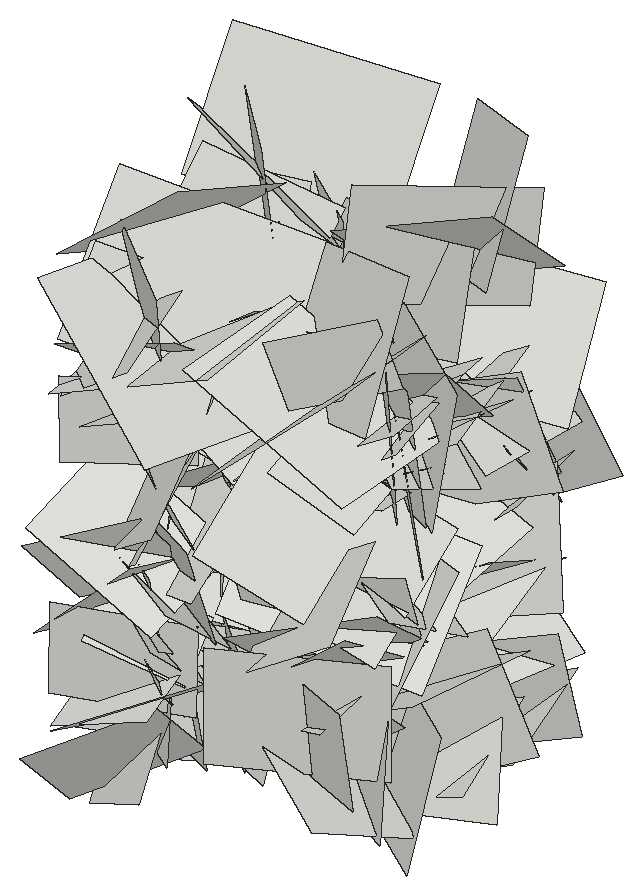
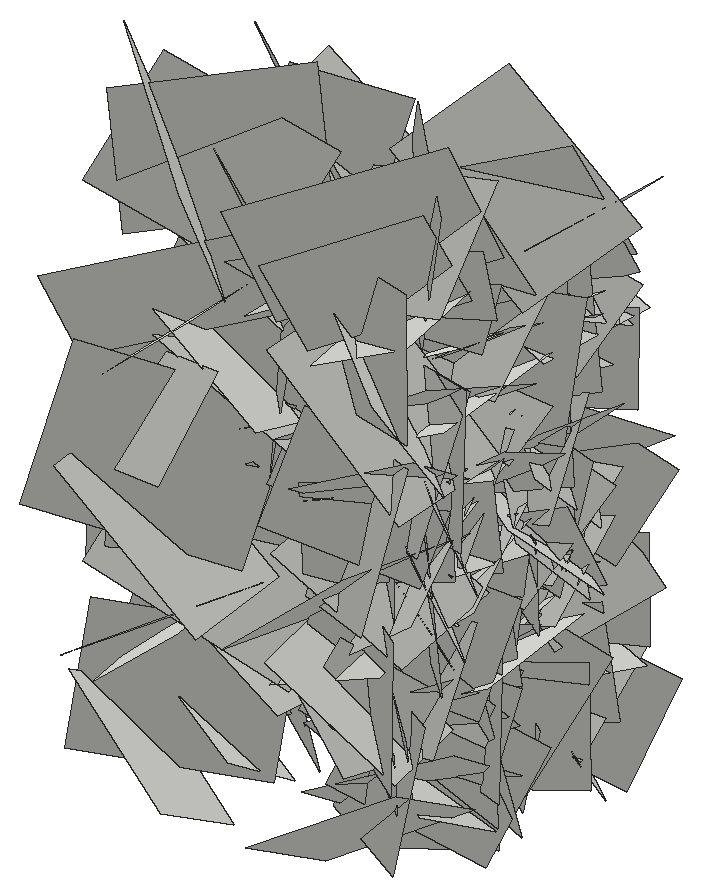
# SketchUp Ruby script. Lengths in inches.
U = 1.inch
M = Sketchup.active_model
def pt(a) = Geom::Point3d.new(a.map { |v| v * U })
def face(e, loops, mat)
  f = e.add_face(loops[0].map { |a| pt(a) })
  loops[1..].each { |l| e.add_face(l.map { |a| pt(a) }).erase! }
  f.material = f.back_material = mat if mat
  f
end
# faces: each face lists its corners as indices into pts; further lists are holes
def faces(e, pts, list, mat = nil) = list.each { |f| face(e, (f[0].is_a?(Array) ? f : [f]).map { |l| l.map { |i| pts[i] } }, mat) }
# xy, xz, yz: faces in a plane at the given z, y or x. An outline is a flat list of corners, or four numbers for a rectangle; further outlines are holes
def ring(l) = l.size == 4 ? [[l[0], l[1]], [l[2], l[1]], [l[2], l[3]], [l[0], l[3]]] : l.each_slice(2).to_a
def flat(e, list, mat, &to3) = list.each { |f| face(e, (f[0].is_a?(Array) ? f : [f]).map { |l| ring(l).map { |u, v| to3.(u, v) } }, mat) }
def xy(e, z, list, mat = nil) = flat(e, list, mat) { |x, y| [x, y, z] }
def xz(e, y, list, mat = nil) = flat(e, list, mat) { |x, z| [x, y, z] }
def yz(e, x, list, mat = nil) = flat(e, list, mat) { |y, z| [x, y, z] }
def lines(e, pts, list) = list.each { |a, b| e.add_line(pt(pts[a]), pt(pts[b])) }
# prism: a flat outline (further loops are holes) pulled along v
def prism(e, loops, v, mat = nil)
  f = face(e, loops, mat); d = Geom::Vector3d.new(v.map { |x| x * U })
  f.pushpull(f.normal.samedirection?(d) ? d.length : -d.length)
end
def box(e, o, s, mat = nil) = prism(e, [[o, [o[0] + s[0], o[1], o[2]], [o[0] + s[0], o[1] + s[1], o[2]], [o[0], o[1] + s[1], o[2]]]], [0, 0, s[2]], mat)
def at(x, y, z, deg = 0) = Geom::Transformation.translation(pt([x, y, z])) * Geom::Transformation.rotation(ORIGIN, Z_AXIS, deg.degrees)
def axes(o, x, y, z) = Geom::Transformation.new([*x, 0, *y, 0, *z, 0, *pt(o).to_a, 1])
def part(name) = M.definitions.add(name)
# library, detail: a bought-in or finely detailed component or shape, given as its bounding box
def library(name, o, s) = part(name).tap { |d| box(d.entities, o, s) }
def detail(e, o, s) = box(e.add_group.entities, o, s)
def put(e, d, t, mat = nil) = e.add_instance(d, t).tap { |i| i.material = mat if mat }
def group(e, t, mat = nil) = e.add_group.tap { |g| g.transformation = t; g.material = mat if mat }.entities
root = M.entities
c1 = part("Component\#6")
p = [[0.01,0,0],[0,3.24,4.54],[4.32,3.24,4.54],[4.33,0,0]]
faces(c1.entities,p,[[0,1,2,3]])
put(root,c1,axes([28.31,154.27,5.56],[0.10843,0.64197,-0.78685],[0.13439,-0.79271,-0.63027],[-1.06801,-0.03458,-0.15919]))
put(root,c1,axes([24.34,149.67,1.32],[0.10197,-0.47157,-0.58691],[-0.00963,-0.59236,0.47447],[0.798,0.05311,0.08072]))
put(root,c1,axes([24.34,151.77,10.3],[0.00621,-0.04081,-0.81439],[0.02737,-0.814,0.04098],[0.86391,0.02608,0.00455]))
put(root,c1,axes([28.31,158.76,13.54],[0.17018,-0.33172,-0.9968],[0.1229,-0.99662,0.35033],[-1.10678,-0.16167,-0.11436]))
put(root,c1,axes([24.34,155.14,21.07],[-0.01676,0.7943,-0.14622],[0.08914,-0.14383,-0.79043],[0.85145,0.03069,0.07988]))
put(root,c1,axes([28.31,152.55,8.85],[0.17208,0.39932,0.93109],[0.08126,0.93542,-0.41455],[-1.07081,0.13515,0.11817]))
put(root,c1,axes([24.34,155.22,14.18],[-0.0107,0.67836,0.43703],[0.08223,0.43585,-0.67474],[0.8514,-0.03357,0.07066]))
put(root,c1,axes([28.31,154.72,7.86],[-0.01434,-0.12328,-0.7123],[-0.10241,-0.70572,0.12398],[-0.75939,0.0975,-0.00327]))
put(root,c1,axes([24.34,153.88,7.81],[0.12498,-0.19712,-0.75186],[-0.05107,-0.76085,0.19192],[0.82232,-0.01729,0.12619]))
put(root,c1,axes([28.31,156.49,11.61],[0.16435,-0.92659,-0.48849],[0.14398,-0.47186,0.93815],[-1.10094,-0.20004,0.04977]))
put(root,c1,axes([28.31,155.82,10.86],[0.10869,-0.77244,0.23734],[-0.13092,0.22145,0.77409],[-0.8465,-0.13343,-0.08925]))
put(root,c1,axes([24.34,152.8,10.75],[-0.04843,-0.82009,-0.82841],[-0.32646,-0.79109,0.80013],[1.19171,-0.25004,0.18553]))
put(root,c1,axes([24.34,146.53,12.92],[0.03124,-0.05121,0.8385],[-0.00373,0.839,0.05136],[0.89046,0.00531,-0.0292]))
put(root,c1,axes([24.34,155.95,10.68],[0.04823,-0.00518,0.84226],[-0.02844,0.84305,0.00663],[0.89236,0.02715,-0.04531]))
put(root,c1,axes([28.31,154.86,6.54],[0.11481,0.21277,-0.79232],[-0.09254,-0.79167,-0.22453],[-0.86468,0.11298,-0.08117]))
put(root,c1,axes([24.34,147.06,-0.97],[0.01135,-0.66277,0.66685],[-0.09721,0.66298,0.66039],[0.99185,0.07256,0.05709]))
put(root,c1,axes([28.31,155.74,21.65],[0.00825,-0.17983,-0.66547],[-0.14401,-0.65286,0.17483],[-0.71636,0.12918,-0.04281]))
put(root,c1,axes([28.31,153.02,6.56],[-0.04835,0.51462,-0.41299],[-0.10228,-0.41473,-0.50612],[-0.69191,0.02534,0.10368]))
put(root,c1,axes([24.34,149.625,17.57],[0.05592,-0.7816,-0.40589],[-0.0657,-0.4089,0.77935],[0.93124,0.01809,0.07936]))
put(root,c1,axes([24.34,152.46,19.1],[-0.24316,-1.11668,0.32256],[-0.08367,0.34299,1.13127],[1.22923,-0.19755,0.14081]))
put(root,c1,axes([24.34,154.93,13.48],[-0.13332,0.92748,-0.67904],[-0.1887,-0.69057,-0.91025],[1.20375,-0.00553,-0.2179]))
put(root,c1,axes([28.31,155.23,10.47],[0.04155,0.12694,-0.87349],[0.11983,-0.86787,-0.12105],[-0.92792,-0.10639,-0.05475]))
put(root,c1,axes([24.34,153.68,-0.24],[0.08313,-0.05331,0.78078],[0.05564,0.78328,0.04821],[0.82769,-0.0473,-0.08166]))
put(root,c1,axes([28.31,152.53,7.1875],[-0.08757,-0.64703,0.3684],[0.09594,0.35919,0.65114],[-0.78338,0.11632,0.03856]))
put(root,c1,axes([28.31,154.48,3.89],[-0.11783,0.23417,0.69133],[0.11259,0.69704,-0.21902],[-0.76547,0.06648,-0.13863]))
put(root,c1,axes([24.34,151.57,3.27],[0.14157,0.02397,-0.74069],[0.04702,-0.75154,-0.01632],[0.78414,0.04073,0.1347]))
put(root,c1,axes([28.31,146.09,12.1875],[0.18427,0.52878,-0.65011],[-0.11203,-0.64482,-0.55274],[-0.8812,0.19255,-0.06567]))
put(root,c1,axes([24.34,147.21,13.43],[-0.06341,1.09172,0.23851],[-0.19798,0.22572,-1.08003],[1.16785,0.09755,-0.17015]))
put(root,c1,axes([28.31,145.53,10.42],[0.22479,1.04725,-0.16356],[0.16331,-0.19548,-1.05191],[-1.11161,0.18306,-0.18761]))
put(root,c1,axes([24.34,149.03,14.67],[-0.12882,0.64149,-0.81464],[0.00451,-0.8199,-0.64626],[1.09909,0.07855,-0.09282]))
put(root,c1,axes([28.31,155.43,2.74],[-0.05213,0.12024,0.7107],[0.06472,0.71048,-0.11598],[-0.7613,0.05216,-0.05853]))
put(root,c1,axes([24.34,146.38,17.95],[0.09245,0.38694,0.78979],[-0.04684,0.79459,-0.38441],[0.93107,0.00155,-0.09776]))
put(root,c1,axes([28.31,155.07,5.6],[0.26442,-0.95782,0.42161],[0.12666,0.45666,0.96674],[-1.10204,-0.17733,0.21227]))
put(root,c1,axes([28.31,154.81,5.31],[-0.03271,-0.68931,-0.29186],[0.0897,-0.29345,0.68411],[-0.78838,-0.00479,0.08995]))
put(root,c1,axes([28.31,148.44,10.1],[-0.02371,0.59128,0.15103],[-0.13632,0.14317,-0.57956],[-0.63236,-0.05303,0.11928]))
put(root,c1,axes([24.34,154.73,4.99],[-0.23466,-0.21907,1.02966],[0.17179,1.03255,0.25453],[1.10257,-0.20751,0.17949]))
put(root,c1,axes([24.34,152.28,1.18],[-0.22482,-0.75958,0.923],[-0.06114,0.94282,0.76264],[1.2656,-0.08938,0.2008]))
put(root,c1,axes([28.31,146.72,8.375],[-0.05548,0.31048,0.67068],[0.12303,0.66747,-0.29994],[-0.77368,0.08387,-0.09579]))
put(root,c1,axes([24.34,147.71,9.53],[-0.0202,0.73421,-0.62443],[0.01239,-0.62433,-0.73445],[1.02159,0.02209,-0.00344]))
put(root,c1,axes([28.31,148.39,13.69],[-0.056,0.56116,0.2115],[-0.06403,0.20626,-0.56234],[-0.63244,-0.07057,0.03821]))
put(root,c1,axes([24.34,149.64,15.49],[-0.05397,-0.71515,0.49033],[0.26351,0.45852,0.69456],[0.88054,-0.18105,-0.1778]))
put(root,c1,axes([24.34,157.06,14.03],[-0.04606,-0.47436,-0.98882],[-0.12961,-0.98133,0.47614],[1.15527,-0.12901,0.01399]))
put(root,c1,axes([24.34,159.16,9.85],[-0.13765,0.1916,-1.18129],[-0.14512,-1.1828,-0.17679],[1.2602,-0.11528,-0.14939]))
put(root,c1,axes([24.34,152.91,14.99],[-0.05042,0.65822,-0.8803],[-0.11398,-0.87969,-0.65195],[1.15954,-0.05785,-0.10236]))
put(root,c1,axes([24.34,158.68,8.63],[-0.07829,-0.94373,0.27717],[0.10215,0.26967,0.94388],[1.03759,-0.09775,-0.07202]))
put(root,c1,axes([28.31,147.13,6.96],[0.04816,-0.19283,0.63159],[-0.07038,0.62854,0.19668],[-0.69645,-0.07685,0.0238]))
put(root,c1,axes([24.34,152.6,3.91],[0.02426,0.68313,0.69515],[-0.0107,0.69547,-0.68312],[1.03305,-0.00884,-0.0234]))
put(root,c1,axes([28.31,153.92,20.8125],[-0.01755,0.277,-0.54123],[-0.05617,-0.54003,-0.27476],[-0.64202,0.03967,0.03883]))
put(root,c1,axes([28.31,156.87,7.65],[-0.00449,0.50233,-0.39291],[-0.02578,-0.39276,-0.50188],[-0.67552,0.01165,0.02176]))
put(root,c1,axes([28.31,147.62,1.41],[0.08717,-0.06025,0.7019],[-0.04865,0.70471,0.06586],[-0.74517,-0.05306,0.07781]))
put(root,c1,axes([28.31,151.79,4.27],[0.00282,-0.67031,0.14172],[0.04158,0.14164,0.66918],[-0.72504,0.00552,0.03892]))
put(root,c1,axes([28.31,151.99,2.12],[0.1775,0.68354,0.35821],[-0.06031,0.37649,-0.69181],[-0.81579,0.12089,0.12909]))
put(root,c1,axes([24.34,154.79,8.7],[-0.06507,0.61236,-0.89404],[-0.03144,-0.89608,-0.61173],[1.14823,0.01016,-0.06741]))
put(root,c1,axes([24.34,155.05,20.66],[0.11898,0.43702,0.87755],[-0.10329,0.88388,-0.42771],[1.03402,0.038,-0.1437]))
put(root,c1,axes([24.34,148.76,4.0625],[0.10183,-0.75916,-0.2873],[0.20096,-0.26032,0.75126],[0.83661,0.15493,-0.14549]))
put(root,c1,axes([28.31,151.13,9.12],[0.15296,0.67587,0.31221],[-0.03502,0.32352,-0.68509],[-0.78839,0.11676,0.09101]))
put(root,c1,axes([24.34,158.45,22.43],[-0.19892,0.24365,-1.12098],[0.08242,-1.13056,-0.25875],[1.21318,0.11676,-0.16622]))
put(root,c1,axes([24.34,153.47,7.93],[-0.25077,0.36385,-1.26635],[-0.08689,-1.28818,-0.35481],[1.39394,-0.01484,-0.24993]))
put(root,c1,axes([28.31,151.91,13.09],[0.06029,-0.61389,0.14039],[-0.0496,0.13645,0.61563],[-0.66568,-0.06576,-0.03315]))
put(root,c1,axes([28.31,155.37,8.05],[0.03179,-0.04018,0.69029],[0.07893,0.6871,0.03676],[-0.72868,0.07267,0.03409]))
put(root,c1,axes([28.31,147.25,18.09],[0.11506,-0.20062,0.68841],[0.02156,0.69683,0.19986],[-0.75976,-0.01061,0.10993]))
put(root,c1,axes([28.31,146,16.15],[0.10062,0.63244,0.10884],[-0.07256,0.11937,-0.63396],[-0.67636,0.08128,0.0842]))
put(root,c1,axes([24.34,157.74,11.21],[0.0595,-0.6331,0.72554],[0.06262,0.72766,0.63038],[1.01877,-0.00775,-0.08112]))
put(root,c1,axes([24.34,160.22,19.0625],[-0.13961,-0.68099,-1.03193],[-0.07146,-1.03227,0.68982],[1.30861,-0.12902,-0.07242]))
put(root,c1,axes([28.31,149.02,5.32],[0.19432,-0.67994,0.40742],[0.04988,0.42677,0.69106],[-0.83874,-0.13215,0.13549]))
put(root,c1,axes([24.34,154.9,1.8],[0.03269,0.90387,0.50014],[0.00572,0.50021,-0.90434],[1.09498,-0.0296,-0.01021]))
put(root,c1,axes([28.31,152.72,13.34],[0.14332,-0.62648,-0.12325],[-0.10799,-0.14554,0.62801],[-0.66813,-0.11086,-0.12794]))
put(root,c1,axes([24.34,157.43,12.97],[-0.1074,-0.05602,-1.35571],[-0.22854,-1.34155,0.07155],[1.42001,-0.22014,-0.09102]))
put(root,c1,axes([24.34,151.01,19.39],[0.01021,0.65154,-0.69294],[0.23408,-0.67557,-0.63214],[0.98066,0.15447,0.1581]))
put(root,c1,axes([24.34,148.31,17.26],[0.09379,0.98835,0.28145],[-0.01751,0.28383,-0.99149],[1.08916,-0.08054,-0.04018]))
put(root,c1,axes([24.34,155.4,17.52],[-0.19723,0.3027,-1.19403],[0.0763,-1.20284,-0.31615],[1.30348,0.11621,-0.16216]))
put(root,c1,axes([24.34,145.87,3.84],[0.08046,-0.07863,0.91675],[0.19442,0.90269,0.06223],[0.95574,-0.17701,-0.08983]))
put(root,c1,axes([24.34,148.09,7.11],[-0.15706,0.67864,1.02073],[0.03183,1.02986,-0.68036],[1.29889,0.05683,0.1401]))
put(root,c1,axes([24.34,148.93,-0.125],[-0.17085,0.2332,1.25619],[-0.02467,1.2654,-0.2379],[1.35409,0.05247,0.15416]))
put(root,c1,axes([24.34,158.83,13.98],[0.00743,-1.2386,0.03478],[-0.17851,0.0335,1.22715],[1.30124,0.01167,0.16814]))
put(root,c1,axes([24.34,152.08,1.74],[0.04493,0.85391,0.54577],[0.09586,0.54089,-0.85328],[1.06994,-0.08432,0.05353]))
put(root,c1,axes([24.34,151.75,19.45],[0.16935,0.44212,0.83371],[0.05466,0.84022,-0.45546],[0.99881,-0.12095,-0.11643]))
put(root,c1,axes([28.31,150.18,6.375],[0.17639,-0.58204,-0.33942],[-0.00316,-0.35025,0.59915],[-0.71419,-0.1422,-0.08648]))
put(root,c1,axes([28.31,148.65,3.04],[0.12439,-0.47488,0.46679],[0.05284,0.47892,0.47469],[-0.70386,-0.04797,0.11813]))
put(root,c1,axes([24.34,156.6875,24.44],[0.16473,0.01802,-1.18121],[-0.23771,-1.16927,-0.04735],[1.22945,-0.22849,0.14911]))
put(root,c1,axes([24.34,147.43,1.76],[0.0449,0.15818,1.07958],[0.0304,1.07985,-0.15935],[1.15617,-0.03454,-0.03773]))
put(root,c1,axes([24.34,158.38,15.93],[-0.03304,0.59909,-1.16183],[-0.1621,-1.15585,-0.5919],[1.37611,-0.12177,-0.09762]))
put(root,c1,axes([24.34,156.09,10.89],[0.02844,-1.01096,-0.23497],[0.17327,-0.228,0.99963],[1.08645,0.06282,-0.15327]))
put(root,c1,axes([24.34,159.05,4.5],[0.22831,-0.97739,-0.02602],[-0.01319,-0.02938,1.00067],[1.03632,0.21495,0.01847]))
put(root,c1,axes([24.34,157.5,5.99],[0.02733,0.34478,-1.12821],[-0.04378,-1.12752,-0.34552],[1.24973,-0.04704,0.01257]))
put(root,c1,axes([24.34,147.25,11.15],[0.01251,0.83252,-0.66438],[0.16644,-0.65852,-0.82239],[1.1167,0.08883,0.13002]))
put(root,c1,axes([28.31,155.94,6.59],[0.14653,0.65267,0.04592],[0.0729,0.03218,-0.6644],[-0.6897,0.14207,-0.06047]))
put(root,c1,axes([24.34,153.16,13.74],[0.07693,-1.07175,0.44962],[-0.07215,0.4458,1.07364],[1.22986,0.09319,0.03486]))
put(root,c1,axes([24.34,150.33,13.2],[-0.24126,0.02501,1.36725],[0.05252,1.3853,-0.01709],[1.44858,-0.04606,0.22834]))
put(root,c1,axes([24.34,144.59,11.1],[0.20686,0.83944,0.54314],[0.00436,0.55271,-0.85571],[1.05982,-0.16612,-0.10249]))
put(root,c1,axes([24.34,153.72,24.55],[-0.10736,0.8301,-0.78481],[0.26067,-0.75358,-0.8288],[1.18252,0.24148,0.11144]))
put(root,c1,axes([24.34,148.8125,12.02],[0.02959,0.36254,-1.01381],[0.21176,-0.99828,-0.35148],[1.12146,0.17893,0.09312]))
put(root,c1,axes([24.34,148.37,14.37],[0.13394,0.02599,1.3483],[-0.3112,1.32226,0.00203],[1.39518,0.29244,-0.12899]))
put(root,c1,axes([24.34,151.84,12.71],[0.09641,-0.969,-0.91768],[-0.24854,-0.9171,0.94515],[1.39265,-0.09659,0.2322]))
put(root,c1,axes([24.34,152.41,8.09],[-0.02535,-1.06677,0.60381],[0.0625,0.60222,1.06631],[1.29785,-0.04984,-0.03955]))
put(root,c1,axes([24.34,153.41,21.56],[0.04666,0.60871,1.19242],[-0.17987,1.18598,-0.59916],[1.40769,0.13136,-0.11609]))
put(root,c1,axes([24.34,154.4,5.48],[-0.14525,-0.2612,-1.20099],[0.27145,-1.18798,0.22915],[1.27422,0.2233,-0.18571]))
put(root,c1,axes([24.34,153.21,11.43],[-0.14123,-0.96535,-0.93141],[0.15435,-0.94087,0.95433],[1.41351,0.00629,-0.19727]))
put(root,c1,axes([24.34,157.09,9.16],[0.26081,-0.66319,-0.77037],[0.09697,-0.77495,0.69635],[1.07312,0.23121,0.12431]))
put(root,c1,axes([24.34,149.27,6.59],[-0.15688,1.33929,-0.00269],[0.18956,0.01708,-1.33541],[1.40693,0.14704,0.17962]))
put(root,c1,axes([24.34,149.82,11.51],[0.16938,-0.10345,1.35904],[-0.25816,1.34416,0.13095],[1.4215,0.25644,-0.13816]))
put(root,c1,axes([24.34,155.16,12.125],[0.20792,1.23942,0.0793],[-0.14973,0.10203,-1.24521],[1.30793,-0.18535,-0.15516]))
put(root,c1,axes([24.34,151.77,16.16],[0.14743,1.12249,0.38129],[0.0578,0.37744,-1.13105],[1.25528,-0.14922,0.00729]))
put(root,c1,axes([24.34,145.22,20.96],[0.20751,1.35949,-0.09859],[-0.20583,-0.07077,-1.36145],[1.43011,-0.20745,-0.18164]))
put(root,c1,axes([24.34,149.47,1.18],[0.22795,-1.08393,0.44752],[0.03192,0.45993,1.09954],[1.24263,0.18702,-0.11034]))
put(root,c1,axes([24.34,155.15,17.37],[0.02517,0.60882,-1.16754],[0.2041,-1.15679,-0.59929],[1.38075,0.1599,0.10987]))
put(root,c1,axes([24.34,146.56,18.67],[0.08115,0.67304,1.19325],[0.03541,1.19384,-0.67552],[1.45175,-0.06674,-0.05023]))
put(root,c1,axes([24.34,150.46,17.01],[0.04698,1.34267,-0.16756],[0.13374,-0.17102,-1.33703],[1.42802,-0.02815,0.13073]))
put(root,c1,axes([24.34,150.02,13.53],[0.11354,-0.10924,1.28227],[0.18202,1.27641,0.09439],[1.35193,-0.16268,-0.1204]))
put(root,c1,axes([24.34,153.54,10.59],[0.17173,1.22834,-0.55665],[0.01226,-0.5619,-1.23655],[1.42944,-0.14275,0.07748]))
put(root,c1,axes([24.34,151.36,16.73],[0.05564,-1.33407,-0.12972],[0.26745,-0.11766,1.31218],[1.39538,0.07575,-0.24633]))
put(root,c1,axes([24.34,148.21,18.05],[0.18781,1.38239,0.05917],[0.11095,0.04609,-1.39025],[1.46247,-0.18102,0.09787]))
put(root,c1,axes([38.11,148.21,18.05],[-0.18781,1.38239,0.05917],[-0.11095,0.04609,-1.39025],[-1.46247,-0.18102,0.09787]))
put(root,c1,axes([38.11,151.36,16.73],[-0.05564,-1.33407,-0.12972],[-0.26745,-0.11766,1.31218],[-1.39538,0.07575,-0.24633]))
put(root,c1,axes([38.11,153.54,10.59],[-0.17173,1.22834,-0.55665],[-0.01226,-0.5619,-1.23655],[-1.42944,-0.14275,0.07748]))
put(root,c1,axes([38.11,150.02,13.53],[-0.11354,-0.10924,1.28227],[-0.18202,1.27641,0.09439],[-1.35193,-0.16268,-0.1204]))
put(root,c1,axes([38.11,150.46,17.01],[-0.04698,1.34267,-0.16756],[-0.13374,-0.17102,-1.33703],[-1.42802,-0.02815,0.13073]))
put(root,c1,axes([38.11,146.56,18.67],[-0.08115,0.67304,1.19325],[-0.03541,1.19384,-0.67552],[-1.45175,-0.06674,-0.05023]))
put(root,c1,axes([38.11,155.15,17.37],[-0.02517,0.60882,-1.16754],[-0.2041,-1.15679,-0.59929],[-1.38075,0.1599,0.10987]))
put(root,c1,axes([38.11,149.47,1.18],[-0.22795,-1.08393,0.44752],[-0.03192,0.45993,1.09954],[-1.24263,0.18702,-0.11034]))
put(root,c1,axes([38.11,145.22,20.96],[-0.20751,1.35949,-0.09859],[0.20583,-0.07077,-1.36145],[-1.43011,-0.20745,-0.18164]))
put(root,c1,axes([38.11,151.77,16.16],[-0.14743,1.12249,0.38129],[-0.0578,0.37744,-1.13105],[-1.25528,-0.14922,0.00729]))
put(root,c1,axes([38.11,155.16,12.125],[-0.20792,1.23942,0.0793],[0.14973,0.10203,-1.24521],[-1.30793,-0.18535,-0.15516]))
put(root,c1,axes([38.11,149.82,11.51],[-0.16938,-0.10345,1.35904],[0.25816,1.34416,0.13095],[-1.4215,0.25644,-0.13816]))
put(root,c1,axes([38.11,149.27,6.59],[0.15688,1.33929,-0.00269],[-0.18956,0.01708,-1.33541],[-1.40693,0.14704,0.17962]))
put(root,c1,axes([38.11,157.09,9.16],[-0.26081,-0.66319,-0.77037],[-0.09697,-0.77495,0.69635],[-1.07312,0.23121,0.12431]))
put(root,c1,axes([38.11,153.21,11.43],[0.14123,-0.96535,-0.93141],[-0.15435,-0.94087,0.95433],[-1.41351,0.00629,-0.19727]))
put(root,c1,axes([38.11,148.05,8.79],[-0.07068,0.0827,-1.14811],[-0.1221,-1.14474,-0.07576],[-1.21402,0.11031,0.07447]))
put(root,c1,axes([38.11,154.4,5.48],[0.14525,-0.2612,-1.20099],[-0.27145,-1.18798,0.22915],[-1.27422,0.2233,-0.18571]))
put(root,c1,axes([38.11,153.41,21.56],[-0.04666,0.60871,1.19242],[0.17987,1.18598,-0.59916],[-1.40769,0.13136,-0.11609]))
put(root,c1,axes([38.11,152.41,8.09],[0.02535,-1.06677,0.60381],[-0.0625,0.60222,1.06631],[-1.29785,-0.04984,-0.03955]))
put(root,c1,axes([38.11,151.84,12.71],[-0.09641,-0.969,-0.91768],[0.24854,-0.9171,0.94515],[-1.39265,-0.09659,0.2322]))
put(root,c1,axes([38.11,148.37,14.37],[-0.13394,0.02599,1.3483],[0.3112,1.32226,0.00203],[-1.39518,0.29244,-0.12899]))
put(root,c1,axes([38.11,148.8125,12.02],[-0.02959,0.36254,-1.01381],[-0.21176,-0.99828,-0.35148],[-1.12146,0.17893,0.09312]))
put(root,c1,axes([38.11,153.72,24.55],[0.10736,0.8301,-0.78481],[-0.26067,-0.75358,-0.8288],[-1.18252,0.24148,0.11144]))
put(root,c1,axes([38.11,144.59,11.1],[-0.20686,0.83944,0.54314],[-0.00436,0.55271,-0.85571],[-1.05982,-0.16612,-0.10249]))
put(root,c1,axes([38.11,150.33,13.2],[0.24126,0.02501,1.36725],[-0.05252,1.3853,-0.01709],[-1.44858,-0.04606,0.22834]))
put(root,c1,axes([38.11,153.16,13.74],[-0.07693,-1.07175,0.44962],[0.07215,0.4458,1.07364],[-1.22986,0.09319,0.03486]))
put(root,c1,axes([34.14,155.94,6.59],[-0.14653,0.65267,0.04592],[-0.0729,0.03218,-0.6644],[0.6897,0.14207,-0.06047]))
put(root,c1,axes([38.11,147.25,11.15],[-0.01251,0.83252,-0.66438],[-0.16644,-0.65852,-0.82239],[-1.1167,0.08883,0.13002]))
put(root,c1,axes([38.11,157.5,5.99],[-0.02733,0.34478,-1.12821],[0.04378,-1.12752,-0.34552],[-1.24973,-0.04704,0.01257]))
put(root,c1,axes([38.11,159.05,4.5],[-0.22831,-0.97739,-0.02602],[0.01319,-0.02938,1.00067],[-1.03632,0.21495,0.01847]))
put(root,c1,axes([38.11,156.09,10.89],[-0.02844,-1.01096,-0.23497],[-0.17327,-0.228,0.99963],[-1.08645,0.06282,-0.15327]))
put(root,c1,axes([38.11,158.38,15.93],[0.03304,0.59909,-1.16183],[0.1621,-1.15585,-0.5919],[-1.37611,-0.12177,-0.09762]))
put(root,c1,axes([38.11,147.43,1.76],[-0.0449,0.15818,1.07958],[-0.0304,1.07985,-0.15935],[-1.15617,-0.03454,-0.03773]))
put(root,c1,axes([38.11,156.6875,24.44],[-0.16473,0.01802,-1.18121],[0.23771,-1.16927,-0.04735],[-1.22945,-0.22849,0.14911]))
put(root,c1,axes([34.14,148.65,3.04],[-0.12439,-0.47488,0.46679],[-0.05284,0.47892,0.47469],[0.70386,-0.04797,0.11813]))
put(root,c1,axes([34.14,150.18,6.375],[-0.17639,-0.58204,-0.33942],[0.00316,-0.35025,0.59915],[0.71419,-0.1422,-0.08648]))
put(root,c1,axes([38.11,151.75,19.45],[-0.16935,0.44212,0.83371],[-0.05466,0.84022,-0.45546],[-0.99881,-0.12095,-0.11643]))
put(root,c1,axes([38.11,152.08,1.74],[-0.04493,0.85391,0.54577],[-0.09586,0.54089,-0.85328],[-1.06994,-0.08432,0.05353]))
put(root,c1,axes([38.11,158.83,13.98],[-0.00743,-1.2386,0.03478],[0.17851,0.0335,1.22715],[-1.30124,0.01167,0.16814]))
put(root,c1,axes([38.11,148.93,-0.125],[0.17085,0.2332,1.25619],[0.02467,1.2654,-0.2379],[-1.35409,0.05247,0.15416]))
put(root,c1,axes([38.11,148.09,7.11],[0.15706,0.67864,1.02073],[-0.03183,1.02986,-0.68036],[-1.29889,0.05683,0.1401]))
put(root,c1,axes([38.11,145.87,3.84],[-0.08046,-0.07863,0.91675],[-0.19442,0.90269,0.06223],[-0.95574,-0.17701,-0.08983]))
put(root,c1,axes([38.11,155.4,17.52],[0.19723,0.3027,-1.19403],[-0.0763,-1.20284,-0.31615],[-1.30348,0.11621,-0.16216]))
put(root,c1,axes([38.11,148.31,17.26],[-0.09379,0.98835,0.28145],[0.01751,0.28383,-0.99149],[-1.08916,-0.08054,-0.04018]))
put(root,c1,axes([38.11,151.01,19.39],[-0.01021,0.65154,-0.69294],[-0.23408,-0.67557,-0.63214],[-0.98066,0.15447,0.1581]))
put(root,c1,axes([38.11,157.43,12.97],[0.1074,-0.05602,-1.35571],[0.22854,-1.34155,0.07155],[-1.42001,-0.22014,-0.09102]))
put(root,c1,axes([34.14,152.72,13.34],[-0.14332,-0.62648,-0.12325],[0.10799,-0.14554,0.62801],[0.66813,-0.11086,-0.12794]))
put(root,c1,axes([38.11,154.9,1.8],[-0.03269,0.90387,0.50014],[-0.00572,0.50021,-0.90434],[-1.09498,-0.0296,-0.01021]))
put(root,c1,axes([34.14,149.02,5.32],[-0.19432,-0.67994,0.40742],[-0.04988,0.42677,0.69106],[0.83874,-0.13215,0.13549]))
put(root,c1,axes([38.11,160.22,19.0625],[0.13961,-0.68099,-1.03193],[0.07146,-1.03227,0.68982],[-1.30861,-0.12902,-0.07242]))
put(root,c1,axes([38.11,157.74,11.21],[-0.0595,-0.6331,0.72554],[-0.06262,0.72766,0.63038],[-1.01877,-0.00775,-0.08112]))
put(root,c1,axes([34.14,146,16.15],[-0.10062,0.63244,0.10884],[0.07256,0.11937,-0.63396],[0.67636,0.08128,0.0842]))
put(root,c1,axes([34.14,147.25,18.09],[-0.11506,-0.20062,0.68841],[-0.02156,0.69683,0.19986],[0.75976,-0.01061,0.10993]))
put(root,c1,axes([34.14,155.37,8.05],[-0.03179,-0.04018,0.69029],[-0.07893,0.6871,0.03676],[0.72868,0.07267,0.03409]))
put(root,c1,axes([34.14,151.91,13.09],[-0.06029,-0.61389,0.14039],[0.0496,0.13645,0.61563],[0.66568,-0.06576,-0.03315]))
put(root,c1,axes([38.11,153.47,7.93],[0.25077,0.36385,-1.26635],[0.08689,-1.28818,-0.35481],[-1.39394,-0.01484,-0.24993]))
